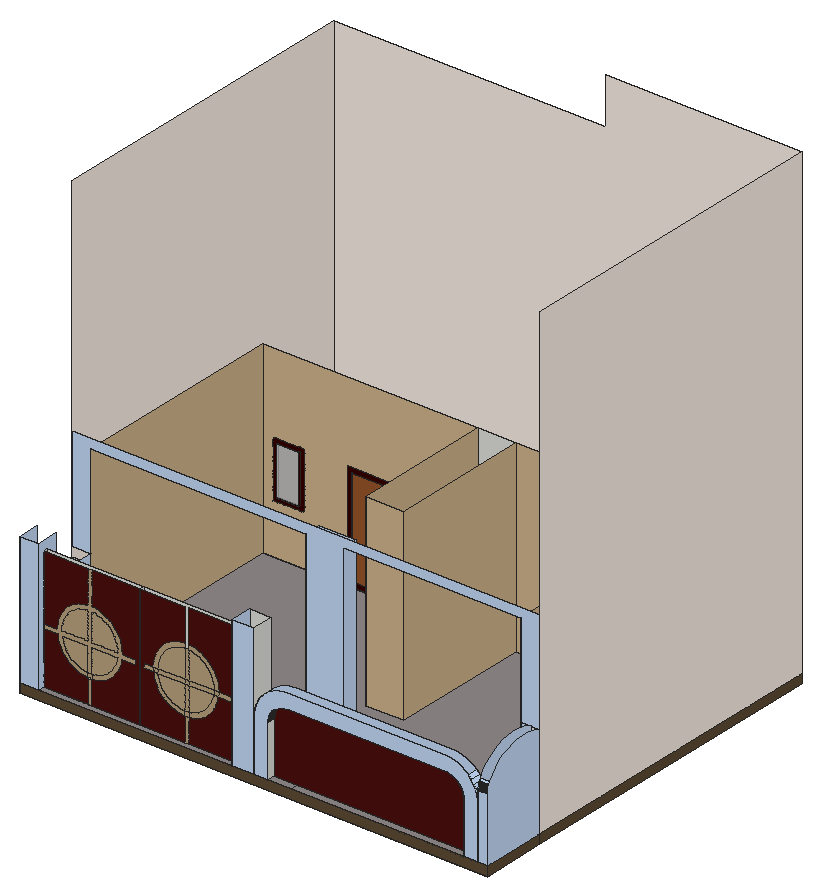
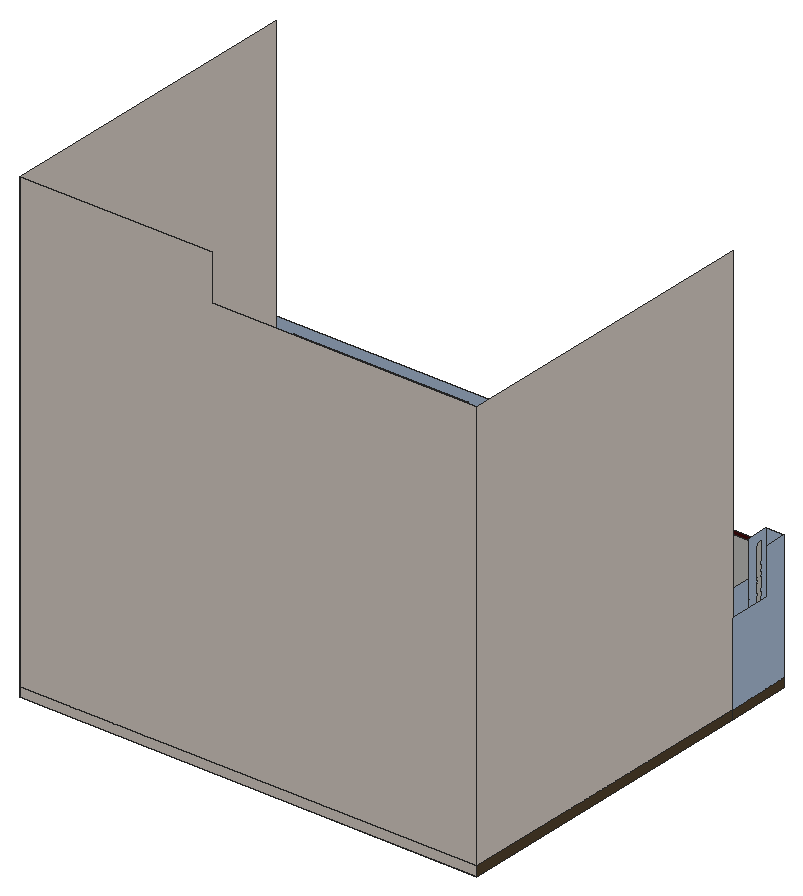
# SketchUp Ruby script. Lengths in inches.
U = 1.inch
M = Sketchup.active_model
def pt(a) = Geom::Point3d.new(a.map { |v| v * U })
def face(e, loops, mat)
  f = e.add_face(loops[0].map { |a| pt(a) })
  loops[1..].each { |l| e.add_face(l.map { |a| pt(a) }).erase! }
  f.material = f.back_material = mat if mat
  f
end
# faces: each face lists its corners as indices into pts; further lists are holes
def faces(e, pts, list, mat = nil) = list.each { |f| face(e, (f[0].is_a?(Array) ? f : [f]).map { |l| l.map { |i| pts[i] } }, mat) }
# xy, xz, yz: faces in a plane at the given z, y or x. An outline is a flat list of corners, or four numbers for a rectangle; further outlines are holes
def ring(l) = l.size == 4 ? [[l[0], l[1]], [l[2], l[1]], [l[2], l[3]], [l[0], l[3]]] : l.each_slice(2).to_a
def flat(e, list, mat, &to3) = list.each { |f| face(e, (f[0].is_a?(Array) ? f : [f]).map { |l| ring(l).map { |u, v| to3.(u, v) } }, mat) }
def xy(e, z, list, mat = nil) = flat(e, list, mat) { |x, y| [x, y, z] }
def xz(e, y, list, mat = nil) = flat(e, list, mat) { |x, z| [x, y, z] }
def yz(e, x, list, mat = nil) = flat(e, list, mat) { |y, z| [x, y, z] }
def lines(e, pts, list) = list.each { |a, b| e.add_line(pt(pts[a]), pt(pts[b])) }
# prism: a flat outline (further loops are holes) pulled along v
def prism(e, loops, v, mat = nil)
  f = face(e, loops, mat); d = Geom::Vector3d.new(v.map { |x| x * U })
  f.pushpull(f.normal.samedirection?(d) ? d.length : -d.length)
end
def box(e, o, s, mat = nil) = prism(e, [[o, [o[0] + s[0], o[1], o[2]], [o[0] + s[0], o[1] + s[1], o[2]], [o[0], o[1] + s[1], o[2]]]], [0, 0, s[2]], mat)
def at(x, y, z, deg = 0) = Geom::Transformation.translation(pt([x, y, z])) * Geom::Transformation.rotation(ORIGIN, Z_AXIS, deg.degrees)
def axes(o, x, y, z) = Geom::Transformation.new([*x, 0, *y, 0, *z, 0, *pt(o).to_a, 1])
def part(name) = M.definitions.add(name)
# library, detail: a bought-in or finely detailed component or shape, given as its bounding box
def library(name, o, s) = part(name).tap { |d| box(d.entities, o, s) }
def detail(e, o, s) = box(e.add_group.entities, o, s)
def put(e, d, t, mat = nil) = e.add_instance(d, t).tap { |i| i.material = mat if mat }
def group(e, t, mat = nil) = e.add_group.tap { |g| g.transformation = t; g.material = mat if mat }.entities
root = M.entities
M.materials.add("[0009_Linen]").color = [250, 240, 230]
M.materials.add("[0022_Maroon]").color = [56, 0, 0]
M.materials.add("[0033_NavajoWhite]").color = [209, 182, 141]
M.materials.add("[0033_NavajoWhite]1").color = [188, 164, 128]
M.materials.add("[0099_LightSteelBlue]").color = [198, 220, 249]
M.materials.add("[Beadboard]").color = [79, 16, 16]
M.materials.add("[Brick Rough Dark]").color = [94, 77, 53]
M.materials.add("[Stone Marble]").color = [143, 138, 136]
M.materials.add("[Translucent Resin Crush Gray]").color = [184, 184, 184]
M.materials["[Translucent Resin Crush Gray]"].alpha = 0.8
M.materials.add("[Wood Cherry Original]").color = [152, 86, 42]
xy(root,0,[[0,0,600,84],[0,84,600,504]])
xy(root,12,[[0,0,24,84],[272.4375,0,300,27.5625],[300,0,318.3125,0,318.3125,10,348,10,348,13.78,300,13.78],[569.6875,0,588,0,588,13.78,348,13.78,348,10,569.6875,10],[588,0,600,84],
  [24,7.78,148.22,13.78],[148.22,7.78,272.4375,13.78],[0,84,24,504],[300,84,348,104.375],[576,84,600,504],
  [300,180,348,360],[24,360,576,504]])
xy(root,12,[[24,0,272.4375,7.78],[318.3125,0,348,10],[348,0,569.6875,10],[24,13.78,272.4375,13.78,272.4375,27.5625,300,27.5625,300,13.78,348,13.78,348,84,300,84,300,104.375,348,104.375,348,84,576,84,576,360,348,360,348,180,300,180,300,360,24,360],[348,13.78,588,84]],"[Stone Marble]")
xy(root,18,[[137.32,360,188.45,361],[388.21,360,456,361]])
xy(root,81.75,[[42.69,359,71.07,360],[236.63,359,265,360]])
xy(root,101.6875,[[342.64,0,545.36,10]])
xz(root,0,[[0,12,24,180],[272.4375,12,300,180],[300,12,318.3125,12,318.3125,77.36,318.35,78.63,318.45,79.9,318.61,81.16,318.85,82.42,319.14,83.66,319.5,84.875,319.93,86.08,320.42,87.25,320.97,88.4,321.57,89.52,322.24,90.61,322.96,91.66,323.74,92.67,324.5625,93.64,325.4375,94.5625,326.36,95.4375,327.33,96.26,328.34,97.04,329.39,97.76,330.48,98.43,331.6,99.03,332.75,99.58,333.92,100.07,335.125,100.5,336.34,100.86,337.58,101.15,338.84,101.39,340.1,101.55,341.37,101.65,342.64,101.6875,545.36,101.6875,548.53,101.48,551.66,100.86,554.67,99.83,557.52,98.43,560.17,96.66,562.5625,94.5625,564.66,92.17,566.43,89.52,567.83,86.67,568.86,83.66,569.48,80.53,569.6875,77.36,569.6875,12,588,12,588,77.36,587.64,82.92,586.55,88.4,584.75,93.68,582.29,98.68,579.1875,103.32,575.51,107.51,571.32,111.1875,566.68,114.29,561.68,116.75,556.4,118.55,550.92,119.64,545.36,120,342.64,120,340.41,119.94,338.18,119.77,335.97,119.48,333.78,119.07,331.6,118.55,329.46,117.91,327.36,117.17,325.3,116.3125,323.28,115.35,321.32,114.29,319.42,113.12,317.58,111.86,315.81,110.5,314.11,109.05,312.49,107.51,310.95,105.89,309.5,104.19,308.14,102.42,306.88,100.58,305.71,98.68,304.65,96.72,303.6875,94.7,302.83,92.64,302.09,90.54,301.45,88.4,300.93,86.22,300.52,84.03,300.23,81.82,300.06,79.59,300,77.36],[588,12,600,94.34]],"[0099_LightSteelBlue]")
xz(root,0,[[0,0,600,12]],"[Brick Rough Dark]")
xz(root,7.78,[[84.43,0.58,84.49,12,80.89,12,80.82,0.6],[84.65,42.34,84.65,42.36,81.05,42.36]])
xz(root,7.78,[[80.89,12,86.11,12,86.11,42.4,85.44,42.34,84.65,42.34,81.05,42.36,80.89,42.38],[205.44,12,210.33,12,210.33,42.51,208.63,42.34,205.44,42.35],[84.65,42.34,85.44,42.34,86.11,42.4,86.11,48.42,85.16,48.33,81.39,48.35,80.89,48.41,80.89,42.38,81.05,42.36,84.65,42.36],[208.63,42.34,210.33,42.51,210.33,48.53,208.35,48.33,205.44,48.35,205.44,42.35],[205.44,42.35,205.44,48.35,204.58,48.35,200.84,48.76,197.16,49.57,193.58,50.75,190.14,52.3,186.89,54.2,183.85,56.43,181.07,58.97,178.5625,61.78,176.36,64.85,174.5,68.12,172.98,71.57,171.84,75.16,171.07,78.85,171.03,79.24,165.01,79.24,165.14,77.94,166.03,73.64,167.37,69.45,169.14,65.42,171.3125,61.6,173.88,58.03,176.8,54.75,180.05,51.79,183.6,49.1875,187.39,46.97,191.4,45.16,195.57,43.78,199.87,42.84,204.24,42.36],
  [[80.89,42.38,80.89,48.41,77.9,48.74,77.65,48.76,73.97,49.57,70.39,50.75,66.96,52.3,63.7,54.2,60.67,56.43,57.88,58.97,55.375,61.78,53.17,64.85,51.31,68.12,49.79,71.57,48.65,75.16,47.89,78.85,47.85,79.24,80.89,79.24,80.89,48.41,81.39,48.35,85.16,48.33,86.11,48.42,86.11,79.24,119.08,79.24,119,78.47,118.19,74.79,117.01,71.21,115.46,67.77,113.56,64.52,111.33,61.48,108.79,58.7,105.98,56.19,102.92,53.99,99.64,52.125,96.19,50.61,92.6,49.47,88.91,48.7,86.11,48.42,86.11,42.4,89.82,42.77,94.125,43.66,98.3125,45,102.34,46.77,106.16,48.94,109.73,51.51,113.01,54.43,115.97,57.68,118.57,61.23,120.79,65.02,122.6,69.03,123.98,73.2,124.92,77.5,125.11,79.24,143.07,79.24,143.07,84.89,125.42,84.89,125.43,86.26,124.99,90.64,124.1,94.94,122.76,99.13,121,103.16,118.82,106.98,116.25,110.55,113.33,113.83,110.08,116.79,106.54,119.39,102.74,121.61,98.73,123.42,94.56,124.8,90.26,125.74,86.11,126.2,86.11,168,80.89,168,80.89,126.18,77.9,125.88,77.125,125.81,72.82,124.92,68.63,123.58,64.61,121.8125,60.79,119.64,57.22,117.07,53.93,114.15,50.97,110.9,48.37,107.35,46.15,103.56,44.34,99.55,42.96,95.38,42.02,91.08,41.54,86.71,41.53,84.89,24,84.89,24,79.24,41.82,79.24,41.95,77.94,42.85,73.64,44.18,69.45,45.95,65.42,48.125,61.6,50.69,58.03,53.61,54.75,56.87,51.79,60.41,49.1875,64.2,46.97,68.21,45.16,72.38,43.78,76.68,42.84,77.9,42.71],[47.52,84.89,47.53,86.37,47.95,90.11,48.75,93.79,49.93,97.37,51.48,100.81,53.39,104.06,55.62,107.1,58.15,109.88,60.97,112.39,64.03,114.59,67.3,116.45,70.75,117.97,74.34,119.11,77.9,119.85,78.03,119.875,80.89,120.16,80.89,84.89],[86.11,84.89,86.11,120.17,89.29,119.82,92.98,119.01,96.55,117.83,99.99,116.28,103.24,114.375,106.28,112.14,109.0625,109.61,111.57,106.79,113.77,103.73,115.64,100.46,117.15,97.01,118.29,93.42,119.06,89.73,119.43,85.98,119.43,84.89]],[210.33,42.51,213.01,42.77,217.3125,43.66,221.5,45,225.53,46.77,229.34,48.94,232.91,51.51,236.2,54.43,239.16,57.68,241.76,61.23,243.98,65.02,245.79,69.03,247.17,73.2,248.11,77.5,248.3,79.24,242.27,79.24,242.19,78.47,241.38,74.79,240.2,71.21,238.65,67.77,236.75,64.52,234.51,61.48,231.98,58.7,229.16,56.19,226.1,53.99,222.83,52.125,219.38,50.61,215.79,49.47,212.1,48.7,210.33,48.53],[208.35,48.33,210.33,48.53,210.33,79.24,205.44,79.24,205.44,48.35],[204.58,48.35,205.44,48.35,205.44,79.24,171.03,79.24,171.07,78.85,171.84,75.16,172.98,71.57,174.5,68.12,176.36,64.85,178.5625,61.78,181.07,58.97,183.85,56.43,186.89,54.2,190.14,52.3,193.58,50.75,197.16,49.57,200.84,48.76],[80.89,48.41,80.89,79.24,47.85,79.24,47.89,78.85,48.65,75.16,49.79,71.57,51.31,68.12,53.17,64.85,55.375,61.78,57.88,58.97,60.67,56.43,63.7,54.2,66.96,52.3,70.39,50.75,73.97,49.57,77.65,48.76,77.9,48.74],
  [86.11,48.42,88.91,48.7,92.6,49.47,96.19,50.61,99.64,52.125,102.92,53.99,105.98,56.19,108.79,58.7,111.33,61.48,113.56,64.52,115.46,67.77,117.01,71.21,118.19,74.79,119,78.47,119.08,79.24,86.11,79.24],[210.33,48.53,212.1,48.7,215.79,49.47,219.38,50.61,222.83,52.125,226.1,53.99,229.16,56.19,231.98,58.7,234.51,61.48,236.75,64.52,238.65,67.77,240.2,71.21,241.38,74.79,242.19,78.47,242.27,79.24,210.33,79.24],[153.21,79.24,165.01,79.24,164.71,82.32,164.72,84.89,153.21,84.89],[165.01,79.24,171.03,79.24,170.7,82.6,170.71,84.89,164.72,84.89,164.71,82.32],[171.03,79.24,205.44,79.24,205.44,84.89,170.71,84.89,170.7,82.6],
  [205.44,79.24,210.33,84.89],[210.33,79.24,242.27,79.24,242.6,82.21,242.61,84.89,210.33,84.89],[242.27,79.24,248.3,79.24,248.59,81.87,248.61,84.89,242.61,84.89,242.6,82.21],[248.3,79.24,272.4375,79.24,272.4375,84.89,248.61,84.89,248.59,81.87],[47.52,84.89,80.89,84.89,80.89,120.16,78.03,119.875,77.9,119.85,74.34,119.11,70.75,117.97,67.3,116.45,64.03,114.59,60.97,112.39,58.15,109.88,55.62,107.1,53.39,104.06,51.48,100.81,49.93,97.37,48.75,93.79,47.95,90.11,47.53,86.37],
  [86.11,84.89,119.43,84.89,119.43,85.98,119.06,89.73,118.29,93.42,117.15,97.01,115.64,100.46,113.77,103.73,111.57,106.79,109.0625,109.61,106.28,112.14,103.24,114.375,99.99,116.28,96.55,117.83,92.98,119.01,89.29,119.82,86.11,120.17],[164.72,84.89,170.71,84.89,170.72,86.37,171.13,90.11,171.9375,93.79,173.12,97.37,174.67,100.81,176.57,104.06,178.8,107.1,181.34,109.88,184.15,112.39,187.21,114.59,190.49,116.45,193.9375,117.97,197.53,119.11,201.22,119.875,204.97,120.25,205.44,120.25,205.44,126.24,204.6875,126.24,200.3125,125.81,196.01,124.92,191.82,123.58,187.79,121.8125,183.97,119.64,180.4,117.07,177.12,114.15,174.16,110.9,171.56,107.35,169.34,103.56,167.53,99.55,166.15,95.38,165.21,91.08,164.73,86.71],[170.71,84.89,205.44,84.89,205.44,120.25,204.97,120.25,201.22,119.875,197.53,119.11,193.9375,117.97,190.49,116.45,187.21,114.59,184.15,112.39,181.34,109.88,178.8,107.1,176.57,104.06,174.67,100.81,173.12,97.37,171.9375,93.79,171.13,90.11,170.72,86.37],[205.44,84.89,210.33,84.89,210.33,120.05,208.74,120.23,205.44,120.25],[210.33,84.89,242.61,84.89,242.62,85.98,242.25,89.73,241.48,93.42,240.34,97.01,238.82,100.46,236.96,103.73,234.76,106.79,232.25,109.61,229.46,112.14,226.43,114.375,223.18,116.28,219.74,117.83,216.16,119.01,212.48,119.82,210.33,120.05],
  [242.61,84.89,248.61,84.89,248.61,86.26,248.18,90.64,247.29,94.94,245.95,99.13,244.18,103.16,242.01,106.98,239.44,110.55,236.52,113.83,233.27,116.79,229.72,119.39,225.93,121.61,221.92,123.42,217.75,124.8,213.45,125.74,210.33,126.08,210.33,120.05,212.48,119.82,216.16,119.01,219.74,117.83,223.18,116.28,226.43,114.375,229.46,112.14,232.25,109.61,234.76,106.79,236.96,103.73,238.82,100.46,240.34,97.01,241.48,93.42,242.25,89.73,242.62,85.98]],"[0033_NavajoWhite]1")
xz(root,7.78,[[24,12,80.89,12,80.89,42.38,77.9,42.71,76.68,42.84,72.38,43.78,68.21,45.16,64.2,46.97,60.41,49.1875,56.87,51.79,53.61,54.75,50.69,58.03,48.125,61.6,45.95,65.42,44.18,69.45,42.85,73.64,41.95,77.94,41.82,79.24,24,79.24],[86.11,12,148.22,12,148.22,168,86.11,168,86.11,126.2,90.26,125.74,94.56,124.8,98.73,123.42,102.74,121.61,106.54,119.39,110.08,116.79,113.33,113.83,116.25,110.55,118.82,106.98,121,103.16,122.76,99.13,124.1,94.94,124.99,90.64,125.43,86.26,125.42,84.89,143.07,84.89,143.07,79.24,125.11,79.24,124.92,77.5,123.98,73.2,122.6,69.03,120.79,65.02,118.57,61.23,115.97,57.68,113.01,54.43,109.73,51.51,106.16,48.94,102.34,46.77,98.3125,45,94.125,43.66,89.82,42.77,86.11,42.4],[148.22,12,205.44,12,205.44,42.35,204.24,42.36,199.87,42.84,195.57,43.78,191.4,45.16,187.39,46.97,183.6,49.1875,180.05,51.79,176.8,54.75,173.88,58.03,171.3125,61.6,169.14,65.42,167.37,69.45,166.03,73.64,165.14,77.94,165.01,79.24,153.21,79.24,153.21,84.89,164.72,84.89,164.73,86.71,165.21,91.08,166.15,95.38,167.53,99.55,169.34,103.56,171.56,107.35,174.16,110.9,177.12,114.15,180.4,117.07,183.97,119.64,187.79,121.8125,191.82,123.58,196.01,124.92,200.3125,125.81,204.6875,126.24,205.44,126.24,205.44,168,148.22,168],[210.33,12,272.4375,12,272.4375,79.24,248.3,79.24,248.11,77.5,247.17,73.2,245.79,69.03,243.98,65.02,241.76,61.23,239.16,57.68,236.2,54.43,232.91,51.51,229.34,48.94,225.53,46.77,221.5,45,217.3125,43.66,213.01,42.77,210.33,42.51],[24,84.89,41.53,84.89,41.54,86.71,42.02,91.08,42.96,95.38,44.34,99.55,46.15,103.56,48.37,107.35,50.97,110.9,53.93,114.15,57.22,117.07,60.79,119.64,64.61,121.8125,68.63,123.58,72.82,124.92,77.125,125.81,77.9,125.88,80.89,126.18,80.89,168,24,168],
  [248.61,84.89,272.4375,84.89,272.4375,168,210.33,168,210.33,126.08,213.45,125.74,217.75,124.8,221.92,123.42,225.93,121.61,229.72,119.39,233.27,116.79,236.52,113.83,239.44,110.55,242.01,106.98,244.18,103.16,245.95,99.13,247.29,94.94,248.18,90.64,248.61,86.26]],"[Beadboard]")
xz(root,10,[[318.3125,12,569.6875,12,569.6875,77.36,569.48,80.53,568.86,83.66,567.83,86.67,566.43,89.52,564.66,92.17,562.5625,94.5625,560.17,96.66,557.52,98.43,554.67,99.83,551.66,100.86,548.53,101.48,545.36,101.6875,342.64,101.6875,341.37,101.65,340.1,101.55,338.84,101.39,337.58,101.15,336.34,100.86,335.125,100.5,333.92,100.07,332.75,99.58,331.6,99.03,330.48,98.43,329.39,97.76,328.34,97.04,327.33,96.26,326.36,95.4375,325.4375,94.5625,324.5625,93.64,323.74,92.67,322.96,91.66,322.24,90.61,321.57,89.52,320.97,88.4,320.42,87.25,319.93,86.08,319.5,84.875,319.14,83.66,318.85,82.42,318.61,81.16,318.45,79.9,318.35,78.63,318.3125,77.36]],"[Beadboard]")
xz(root,13.78,[[24,12,148.22,168],[148.22,12,272.4375,168]])
xz(root,13.78,[[300,12,300,77.36,300.06,79.59,300.23,81.82,300.52,84.03,300.93,86.22,301.45,88.4,302.09,90.54,302.83,92.64,303.6875,94.7,304.65,96.72,305.71,98.68,306.88,100.58,308.14,102.42,309.5,104.19,310.95,105.89,312.49,107.51,314.11,109.05,315.81,110.5,317.58,111.86,319.42,113.12,321.32,114.29,323.28,115.35,325.3,116.3125,327.36,117.17,329.46,117.91,331.6,118.55,333.78,119.07,335.97,119.48,338.18,119.77,340.41,119.94,342.64,120,545.36,120,550.92,119.64,556.4,118.55,561.68,116.75,566.68,114.29,571.32,111.1875,575.51,107.51,579.1875,103.32,582.29,98.68,584.75,93.68,586.55,88.4,587.64,82.92,588,77.36,588,12]],"[0099_LightSteelBlue]")
xz(root,27.5625,[[272.4375,12,300,180]])
xz(root,84,[[0,12,24,120],[588,12,600,132]])
xz(root,84,[[300,12,348,12,348,252,576,252,576,132,600,132,600,264,0,264,0,132,24,132,24,252,300,252],[576,12,588,132]],"[0099_LightSteelBlue]")
xz(root,104.375,[[300,12,348,252]],"[0099_LightSteelBlue]")
xz(root,180,[[300,12,348,252]],"[0033_NavajoWhite]")
xz(root,359,[[42.69,81.75,71.07,143.8125],[236.63,81.75,265,143.8125]],"[Translucent Resin Crush Gray]")
xz(root,360,[[300,12,348,252]])
xz(root,360,[[[131.32,12,194.45,149.8125],[137.32,18,188.45,143.8125]],[[382.21,12,462,158.24],[388.21,18,456,152.24]],[[36.69,75.75,77.07,149.8125],[42.69,81.75,71.07,143.8125]],[[230.63,75.75,271,149.8125],[236.63,81.75,265,143.8125]]],"[0022_Maroon]")
xz(root,360,[[[24,12,131.32,12,131.32,149.8125,194.45,149.8125,194.45,12,300,12,300,252,24,252],[36.69,75.75,77.07,149.8125],[230.63,75.75,271,149.8125]],[348,12,382.21,12,382.21,158.24,462,158.24,462,12,576,12,576,252,348,252]],"[0033_NavajoWhite]")
xz(root,361,[[137.32,18,188.45,143.8125],[388.21,18,456,152.24]],"[Wood Cherry Original]")
xz(root,504,[[0,0,600,12],[0,12,0,552,348,552,348,612,600,612,600,12]],"[0009_Linen]")
yz(root,0,[[84,12,504,552]],"[0009_Linen]")
yz(root,0,[[0,12,0,180,27.5625,180,27.5625,120,84,120,84,12]],"[0099_LightSteelBlue]")
yz(root,0,[[0,0,84,12],[84,0,504,12]],"[Brick Rough Dark]")
yz(root,24,[[7.78,12,13.78,168]])
yz(root,24,[[84,12,360,252]],"[0033_NavajoWhite]")
yz(root,24,[[0,12,7.78,12,7.78,168,13.78,168,13.78,12,27.5625,12,27.5625,180,0,180],[27.5625,12,84,132]],"[0099_LightSteelBlue]")
yz(root,42.69,[[359,81.75,360,143.8125]])
yz(root,71.07,[[359,81.75,360,143.8125]],"[0022_Maroon]")
yz(root,137.32,[[360,18,361,143.8125]],"[0022_Maroon]")
yz(root,148.22,[[7.78,12,13.78,168]])
yz(root,188.45,[[360,18,361,143.8125]])
yz(root,236.63,[[359,81.75,360,143.8125]])
yz(root,265,[[359,81.75,360,143.8125]])
yz(root,272.4375,[[7.78,12,13.78,168]])
yz(root,272.4375,[[0,12,0,180,27.5625,180,27.5625,12,13.78,12,13.78,168,7.78,168,7.78,12]],"[0099_LightSteelBlue]")
yz(root,300,[[0,12,13.78,77.36],[13.78,12,27.5625,12,27.5625,180,0,180,0,77.36,13.78,77.36]])
yz(root,300,[[180,12,360,252]],"[0033_NavajoWhite]")
yz(root,300,[[84,12,104.375,252]],"[0099_LightSteelBlue]")
yz(root,318.3125,[[0,12,10,77.36]])
yz(root,348,[[180,12,360,252]],"[0033_NavajoWhite]")
yz(root,348,[[84,12,104.375,252]],"[0099_LightSteelBlue]")
yz(root,388.21,[[360,18,361,152.24]])
yz(root,456,[[360,18,361,152.24]])
yz(root,569.6875,[[0,12,10,77.36]])
yz(root,576,[[84,12,360,252]],"[0033_NavajoWhite]")
yz(root,588,[[0,12,13.78,77.36]])
yz(root,588,[[13.78,12,13.78,77.36,0,77.36,0,94.34,0.02,95.44,0.1,96.54,0.22,97.64,0.4,98.73,0.62,99.8,0.89,100.87,1.21,101.93,1.58,102.97,1.99,103.99,2.19,104.42,3.51,106.92,7.87,113.24,12.96,118.98,13.78,119.71,18.7,124.07,25.02,128.43,31.8125,132,40.22,135.09,48.97,136.97,57.91,137.6,66.84,136.97,75.6,135.09,84,132,84,12]],"[0099_LightSteelBlue]")
yz(root,600,[[2.19,104.42,3.51,106.92,2.96,105.97,2.45,104.99]])
yz(root,600,[[84,12,504,612]],"[0009_Linen]")
yz(root,600,[[0,12,84,12,84,132,75.6,135.09,66.84,136.97,57.91,137.6,48.97,136.97,40.22,135.09,31.8125,132,25.02,128.43,18.7,124.07,12.96,118.98,7.87,113.24,3.51,106.92,2.19,104.42,1.99,103.99,1.58,102.97,1.21,101.93,0.89,100.87,0.62,99.8,0.4,98.73,0.22,97.64,0.1,96.54,0.02,95.44,0,94.34]],"[0099_LightSteelBlue]")
yz(root,600,[[0,0,84,12],[84,0,504,12]],"[Brick Rough Dark]")
p = [[300.06,13.78,79.59],[300,13.78,77.36],[300,0,77.36],[300.06,0,79.59],[318.35,0,78.63],[318.3125,0,77.36],
  [318.3125,10,77.36],[318.35,10,78.63],[569.6875,0,77.36],[569.48,0,80.53],[569.48,10,80.53],[569.6875,10,77.36],
  [588,13.78,77.36],[587.64,13.78,82.92],[587.64,0,82.92],[588,0,77.36],[318.45,0,79.9],[318.45,10,79.9],
  [300.23,13.78,81.82],[300.23,0,81.82],[318.61,0,81.16],[318.61,10,81.16],[568.86,0,83.66],[568.86,10,83.66],
  [318.85,0,82.42],[318.85,10,82.42],[300.52,13.78,84.03],[300.52,0,84.03],[319.14,0,83.66],[319.14,10,83.66],
  [586.55,13.78,88.4],[586.55,0,88.4],[319.5,0,84.875],[319.5,10,84.875],[567.83,0,86.67],[567.83,10,86.67],
  [300.93,13.78,86.22],[300.93,0,86.22],[319.93,0,86.08],[319.93,10,86.08],[320.42,0,87.25],[320.42,10,87.25],
  [301.45,13.78,88.4],[301.45,0,88.4],[566.43,0,89.52],[566.43,10,89.52],[320.97,0,88.4],[320.97,10,88.4],
  [302.09,13.78,90.54],[302.09,0,90.54],[321.57,0,89.52],[321.57,10,89.52],[584.75,13.78,93.68],[584.75,0,93.68],
  [322.24,0,90.61],[322.24,10,90.61],[564.66,0,92.17],[564.66,10,92.17],[302.83,13.78,92.64],[302.83,0,92.64],
  [322.96,0,91.66],[322.96,10,91.66],[323.74,0,92.67],[323.74,10,92.67],[562.5625,0,94.5625],[562.5625,10,94.5625],
  [303.6875,13.78,94.7],[303.6875,0,94.7],[324.5625,0,93.64],[324.5625,10,93.64],[325.4375,0,94.5625],[325.4375,10,94.5625],
  [582.29,13.78,98.68],[582.29,0,98.68],[600,0,94.34],[600,0.02,95.44],[588,0.02,95.44],[588,0,94.34],
  [326.36,0,95.4375],[326.36,10,95.4375],[560.17,0,96.66],[560.17,10,96.66],[304.65,13.78,96.72],[304.65,0,96.72],
  [327.33,0,96.26],[327.33,10,96.26],[600,0.1,96.54],[588,0.1,96.54],[328.34,0,97.04],[328.34,10,97.04],
  [600,0.22,97.64],[588,0.22,97.64],[305.71,13.78,98.68],[305.71,0,98.68],[557.52,0,98.43],[557.52,10,98.43],
  [329.39,0,97.76],[329.39,10,97.76],[600,0.4,98.73],[588,0.4,98.73],[330.48,0,98.43],[330.48,10,98.43],
  [331.6,0,99.03],[331.6,10,99.03],[554.67,0,99.83],[554.67,10,99.83],[306.88,13.78,100.58],[306.88,0,100.58],
  [579.1875,13.78,103.32],[579.1875,0,103.32],[600,0.62,99.8],[588,0.62,99.8],[332.75,0,99.58],[332.75,10,99.58],
  [333.92,0,100.07],[333.92,10,100.07],[551.66,0,100.86],[551.66,10,100.86],[600,0.89,100.87],[588,0.89,100.87],
  [335.125,0,100.5],[335.125,10,100.5],[336.34,0,100.86],[336.34,10,100.86],[308.14,13.78,102.42],[308.14,0,102.42],
  [337.58,0,101.15],[337.58,10,101.15],[548.53,0,101.48],[548.53,10,101.48],[600,1.21,101.93],[588,1.21,101.93],
  [338.84,0,101.39],[338.84,10,101.39],[340.1,0,101.55],[340.1,10,101.55],[545.36,0,101.6875],[545.36,10,101.6875],
  [341.37,0,101.65],[341.37,10,101.65],[342.64,0,101.6875],[342.64,10,101.6875],[600,1.58,102.97],[588,1.58,102.97],
  [309.5,13.78,104.19],[309.5,0,104.19],[600,1.99,103.99],[588,1.99,103.99],[575.51,13.78,107.51],[575.51,0,107.51],
  [600,2.19,104.42],[588,2.19,104.42],[310.95,13.78,105.89],[310.95,0,105.89],[600,3.51,106.92],[588,3.51,106.92],
  [312.49,13.78,107.51],[312.49,0,107.51]]
faces(root,p,[[0,1,2,3],[12,13,14,15],[18,0,3,19],[26,18,19,27],[13,30,31,14],[36,26,27,37],[42,36,37,43],[48,42,43,49],
  [30,52,53,31],[58,48,49,59],[66,58,59,67],[52,72,73,53],[74,75,76,77],[82,66,67,83],[75,86,87,76],[86,90,91,87],
  [92,82,83,93],[90,98,99,91],[106,92,93,107],[72,108,109,73],[98,110,111,99],[110,118,119,111],[124,106,107,125],[118,130,131,119],
  [130,142,143,131],[144,124,125,145],[142,146,147,143],[108,148,149,109],[146,150,151,147],[152,144,145,153],[150,154,155,151],[156,152,153,157]],"[0099_LightSteelBlue]")
faces(root,p,[[4,5,6,7],[8,9,10,11],[16,4,7,17],[20,16,17,21],[9,22,23,10],[24,20,21,25],[28,24,25,29],[32,28,29,33],
  [22,34,35,23],[38,32,33,39],[40,38,39,41],[34,44,45,35],[46,40,41,47],[50,46,47,51],[54,50,51,55],[44,56,57,45],
  [60,54,55,61],[62,60,61,63],[56,64,65,57],[68,62,63,69],[70,68,69,71],[78,70,71,79],[64,80,81,65],[84,78,79,85],
  [88,84,85,89],[80,94,95,81],[96,88,89,97],[100,96,97,101],[102,100,101,103],[94,104,105,95],[112,102,103,113],[114,112,113,115],
  [104,116,117,105],[120,114,115,121],[122,120,121,123],[126,122,123,127],[116,128,129,117],[132,126,127,133],[134,132,133,135],[128,136,137,129],
  [138,134,135,139],[140,138,139,141]])
